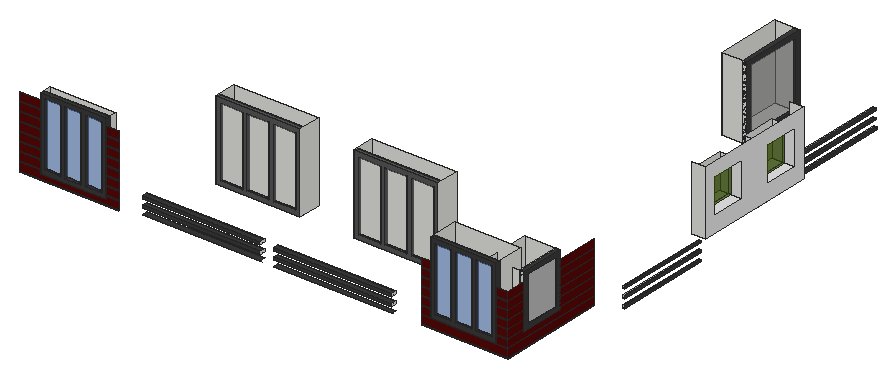
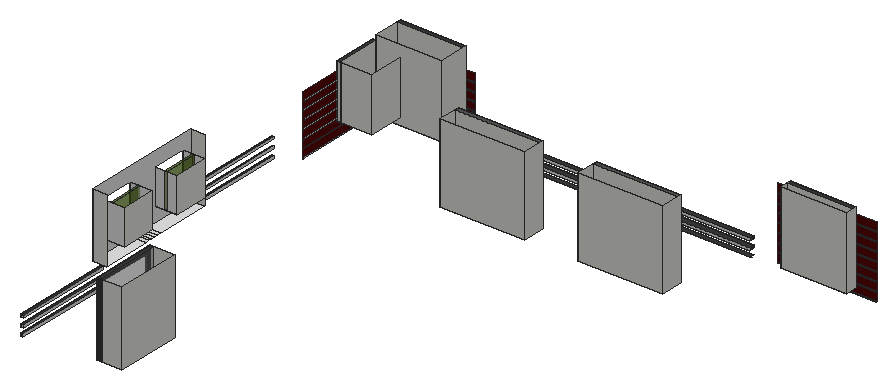
# SketchUp Ruby script. Lengths in inches.
U = 1.inch
M = Sketchup.active_model
def pt(a) = Geom::Point3d.new(a.map { |v| v * U })
def face(e, loops, mat)
  f = e.add_face(loops[0].map { |a| pt(a) })
  loops[1..].each { |l| e.add_face(l.map { |a| pt(a) }).erase! }
  f.material = f.back_material = mat if mat
  f
end
# faces: each face lists its corners as indices into pts; further lists are holes
def faces(e, pts, list, mat = nil) = list.each { |f| face(e, (f[0].is_a?(Array) ? f : [f]).map { |l| l.map { |i| pts[i] } }, mat) }
# xy, xz, yz: faces in a plane at the given z, y or x. An outline is a flat list of corners, or four numbers for a rectangle; further outlines are holes
def ring(l) = l.size == 4 ? [[l[0], l[1]], [l[2], l[1]], [l[2], l[3]], [l[0], l[3]]] : l.each_slice(2).to_a
def flat(e, list, mat, &to3) = list.each { |f| face(e, (f[0].is_a?(Array) ? f : [f]).map { |l| ring(l).map { |u, v| to3.(u, v) } }, mat) }
def xy(e, z, list, mat = nil) = flat(e, list, mat) { |x, y| [x, y, z] }
def xz(e, y, list, mat = nil) = flat(e, list, mat) { |x, z| [x, y, z] }
def yz(e, x, list, mat = nil) = flat(e, list, mat) { |y, z| [x, y, z] }
def lines(e, pts, list) = list.each { |a, b| e.add_line(pt(pts[a]), pt(pts[b])) }
# prism: a flat outline (further loops are holes) pulled along v
def prism(e, loops, v, mat = nil)
  f = face(e, loops, mat); d = Geom::Vector3d.new(v.map { |x| x * U })
  f.pushpull(f.normal.samedirection?(d) ? d.length : -d.length)
end
def box(e, o, s, mat = nil) = prism(e, [[o, [o[0] + s[0], o[1], o[2]], [o[0] + s[0], o[1] + s[1], o[2]], [o[0], o[1] + s[1], o[2]]]], [0, 0, s[2]], mat)
def at(x, y, z, deg = 0) = Geom::Transformation.translation(pt([x, y, z])) * Geom::Transformation.rotation(ORIGIN, Z_AXIS, deg.degrees)
def axes(o, x, y, z) = Geom::Transformation.new([*x, 0, *y, 0, *z, 0, *pt(o).to_a, 1])
def part(name) = M.definitions.add(name)
# library, detail: a bought-in or finely detailed component or shape, given as its bounding box
def library(name, o, s) = part(name).tap { |d| box(d.entities, o, s) }
def detail(e, o, s) = box(e.add_group.entities, o, s)
def put(e, d, t, mat = nil) = e.add_instance(d, t).tap { |i| i.material = mat if mat }
def group(e, t, mat = nil) = e.add_group.tap { |g| g.transformation = t; g.material = mat if mat }.entities
root = M.entities
M.materials.add("Generic").color = [86, 8, 8]
M.materials.add("Generic\#5").color = [230, 230, 230]
M.materials.add("[Color M06]").color = [86, 86, 86]
M.materials.add("[Color M07]").color = [58, 58, 58]
M.materials.add("[Mirror 01]").color = [185, 185, 185]
M.materials.add("[Mirror 02]1").color = [226, 226, 226]
M.materials["[Mirror 02]1"].alpha = 0.26
M.materials.add("[Translucent Glass Blue]").color = [100, 149, 237]
M.materials["[Translucent Glass Blue]"].alpha = 0.5
M.materials.add("[Translucent Glass Dark Green]").color = [62, 91, 5]
M.materials["[Translucent Glass Dark Green]"].alpha = 0.5
M.materials.add("[Translucent Glass Gray]").color = [127, 127, 127]
M.materials["[Translucent Glass Gray]"].alpha = 0.35
c1 = part("Group\#5")
xy(c1.entities,0,[[0,0,6,92.0625]],"[Color M07]")
xy(c1.entities,6.58,[[3,6.58,6,85.48]],"[Color M07]")
xy(c1.entities,96.73,[[3,6.58,6,85.48]],"[Color M07]")
xy(c1.entities,103.3125,[[0,0,6,92.0625]],"[Color M07]")
xz(c1.entities,0,[[0,0,6,103.3125]],"[Color M07]")
xz(c1.entities,6.58,[[3,6.58,6,96.73]],"[Color M07]")
xz(c1.entities,85.48,[[3,6.58,6,96.73]],"[Color M07]")
xz(c1.entities,92.0625,[[0,0,6,103.3125]],"[Color M07]")
yz(c1.entities,0,[[0,0,92.0625,103.3125]],"[Translucent Glass Gray]")
yz(c1.entities,3,[[6.58,6.58,85.48,96.73]],"[Translucent Glass Gray]")
yz(c1.entities,6,[[[0,0,92.0625,103.3125],[6.58,6.58,85.48,96.73]]],"[Color M07]")
c2 = part("Group\#4")
xy(c2.entities,0,[[0,0,117.75,6]],"[Color M06]")
xy(c2.entities,6.37,[[6.37,0,37.125,3],[43.5,0,74.25,3],[80.625,0,111.38,3]],"[Color M06]")
xy(c2.entities,103.75,[[6.37,0,37.125,3],[43.5,0,74.25,3],[80.625,0,111.38,3]],"[Color M06]")
xy(c2.entities,110.125,[[0,0,117.75,6]],"[Color M06]")
xz(c2.entities,0,[[[0,0,117.75,110.125],[6.37,6.37,37.125,103.75],[80.625,6.37,111.38,103.75],[43.5,6.37,74.25,103.75]]],"[Color M06]")
xz(c2.entities,3,[[6.37,6.37,37.125,103.75],[43.5,6.37,74.25,103.75],[80.625,6.37,111.38,103.75]],"[Mirror 02]1")
xz(c2.entities,6,[[0,0,117.75,110.125]])
yz(c2.entities,0,[[0,0,6,110.125]],"[Color M06]")
yz(c2.entities,6.37,[[0,6.37,3,103.75]],"[Color M06]")
yz(c2.entities,37.125,[[0,6.37,3,103.75]],"[Color M06]")
yz(c2.entities,43.5,[[0,6.37,3,103.75]],"[Color M06]")
yz(c2.entities,74.25,[[0,6.37,3,103.75]],"[Color M06]")
yz(c2.entities,80.625,[[0,6.37,3,103.75]],"[Color M06]")
yz(c2.entities,111.38,[[0,6.37,3,103.75]],"[Color M06]")
yz(c2.entities,117.75,[[0,0,6,110.125]],"[Color M06]")
c3 = part("Group\#2")
xy(c3.entities,0,[[0,0,91.6875,6]],"[Color M07]")
xy(c3.entities,6.1,[[6.1,0,28.53,3],[34.63,0,57.06,3],[63.16,0,85.59,3]],"[Color M07]")
xy(c3.entities,95.34,[[6.1,0,28.53,3],[34.63,0,57.06,3],[63.16,0,85.59,3]],"[Color M07]")
xy(c3.entities,101.4375,[[0,0,91.6875,6]],"[Color M07]")
xz(c3.entities,0,[[[0,0,91.6875,101.4375],[34.63,6.1,57.06,95.34],[63.16,6.1,85.59,95.34],[6.1,6.1,28.53,95.34]]],"[Color M07]")
xz(c3.entities,3,[[6.1,6.1,28.53,95.34],[34.63,6.1,57.06,95.34],[63.16,6.1,85.59,95.34]],"[Translucent Glass Blue]")
xz(c3.entities,6,[[0,0,91.6875,101.4375]])
yz(c3.entities,0,[[0,0,6,101.4375]],"[Color M07]")
yz(c3.entities,6.1,[[0,6.1,3,95.34]],"[Color M07]")
yz(c3.entities,28.53,[[0,6.1,3,95.34]],"[Color M07]")
yz(c3.entities,34.63,[[0,6.1,3,95.34]],"[Color M07]")
yz(c3.entities,57.06,[[0,6.1,3,95.34]],"[Color M07]")
yz(c3.entities,63.16,[[0,6.1,3,95.34]],"[Color M07]")
yz(c3.entities,85.59,[[0,6.1,3,95.34]],"[Color M07]")
yz(c3.entities,91.6875,[[0,0,6,101.4375]],"[Color M07]")
c4 = part("Group\#3")
xy(c4.entities,0,[[0,0,6,62.6875]],"[Color M07]")
xy(c4.entities,6.1,[[3,6.1,6,56.59]],"[Color M07]")
xy(c4.entities,69.52,[[3,6.1,6,56.59]],"[Color M07]")
xy(c4.entities,75.625,[[0,0,6,62.6875]],"[Color M07]")
xz(c4.entities,0,[[0,0,6,75.625]],"[Color M07]")
xz(c4.entities,6.1,[[3,6.1,6,69.52]],"[Color M07]")
xz(c4.entities,56.59,[[3,6.1,6,69.52]],"[Color M07]")
xz(c4.entities,62.6875,[[0,0,6,75.625]],"[Color M07]")
yz(c4.entities,0,[[0,0,62.6875,75.625]])
yz(c4.entities,3,[[6.1,6.1,56.59,69.52]],"[Mirror 01]")
yz(c4.entities,6,[[[0,0,62.6875,75.625],[6.1,6.1,56.59,69.52]]],"[Color M07]")
c5 = part("Group\#1")
box(c5.entities,[0,0,0],[3,48.3125,48.3125],"[Translucent Glass Dark Green]")
xy(root,651.9375,[[16.6875,113.625,154.5,113.92]])
xy(root,652.65,[[563.75,654.65,598.75,746.71]])
xy(root,652.9375,[[16.6875,113.625,154.5,113.92]])
xy(root,653.82,[[367.1875,118.5,531.5625,125.9375]],"[Color M07]")
xy(root,654.54,[[183.5625,118.5,347.9375,125.9375]],"[Color M07]")
xy(root,656.21,[[205.11,219.4375,322.86,251.5625],[397.99,219.4375,515.74,251.5625]])
xy(root,656.79,[[723.95,281.625,727.32,413.625]],"[Color M07]")
xy(root,656.83,[[689.08,624.8125,693.27,762.8125]],"[Color M07]")
xy(root,657.48,[[577.6875,113.625,698.4375,113.92],[698.14,113.92,698.4375,263.625]])
xy(root,658.48,[[577.6875,113.625,698.4375,113.92],[698.14,113.92,698.4375,263.625]])
xy(root,659.61,[[44.83,113.625,136.51,130.0625]])
xy(root,659.92,[[723.95,281.625,727.32,413.625]],"[Color M07]")
xy(root,660.15,[[689.08,624.8125,693.27,762.8125]],"[Color M07]")
xy(root,662,[[367.1875,118.5,531.5625,125.9375]],"[Color M07]")
xy(root,662.73,[[183.5625,118.5,347.9375,125.9375]],"[Color M07]")
xy(root,664.4375,[[16.6875,113.625,44.83,113.625,44.83,113.93,16.6875,113.92],[136.51,113.625,154.5,113.625,154.5,113.92,136.51,113.93]])
xy(root,665.4375,[[16.6875,113.625,16.6875,113.92,44.83,113.93,44.83,113.625],[136.51,113.625,136.51,113.93,154.5,113.92,154.5,113.625]])
xy(root,665.82,[[367.1875,118.5,531.5625,125.9375]],"[Color M07]")
xy(root,666.54,[[183.5625,118.5,347.9375,125.9375]],"[Color M07]")
xy(root,668.79,[[723.95,281.625,727.32,413.625]],"[Color M07]")
xy(root,668.8125,[[688.37,624.8125,692.56,762.8125]],"[Color M07]")
xy(root,669.42,[[577.6875,113.625,698.4375,113.92],[698.14,113.92,698.4375,263.625]])
xy(root,669.93,[[589.83,113.93,681.51,156.125]])
xy(root,670.42,[[577.6875,113.625,577.6875,113.92,589.83,113.93,589.83,113.625],[681.51,113.625,681.51,113.93,698.14,113.92,698.4375,113.92,698.4375,113.625],[698.14,113.92,698.4375,263.625]])
xy(root,671.92,[[723.95,281.625,727.32,413.625]],"[Color M07]")
xy(root,672.125,[[688.37,624.8125,692.56,762.8125]],"[Color M07]")
xy(root,672.98,[[698.4375,510.93,717.1875,516.93],[698.4375,516.93,717.1875,521.18],[698.4375,521.18,717.1875,527.18],[698.4375,527.18,717.1875,531.45],[698.4375,531.45,717.1875,537.45]])
xy(root,672.98,[[698.4375,434.68,717.1875,510.93],[698.4375,537.45,717.1875,606.05]],"Generic\#5")
xy(root,674,[[367.1875,118.5,531.5625,125.9375]],"[Color M07]")
xy(root,674.73,[[183.5625,118.5,347.9375,125.9375]],"[Color M07]")
xy(root,676.9375,[[16.6875,113.625,44.83,113.625,44.83,113.93,16.6875,113.92],[136.51,113.625,154.5,113.625,154.5,113.92,136.51,113.93]])
xy(root,677.82,[[367.1875,118.5,531.5625,125.9375]],"[Color M07]")
xy(root,677.9375,[[16.6875,113.625,16.6875,113.92,44.83,113.93,44.83,113.625],[136.51,113.625,136.51,113.93,154.5,113.92,154.5,113.625]])
xy(root,678.54,[[183.5625,118.5,347.9375,125.9375]],"[Color M07]")
xy(root,678.61,[[648.625,141.33,698.4375,204.02]])
xy(root,680.79,[[723.95,281.625,727.32,413.625]],"[Color M07]")
xy(root,680.8125,[[688.37,624.8125,692.56,762.8125]],"[Color M07]")
xy(root,681.37,[[577.6875,113.625,589.83,113.625,589.83,113.93,577.6875,113.92],[681.51,113.625,698.4375,113.625,698.4375,113.92,698.14,113.92,681.51,113.93],[698.14,113.92,698.4375,141.33]])
xy(root,681.72,[[698.14,204.02,698.4375,263.625]])
xy(root,682.37,[[577.6875,113.625,577.6875,113.92,589.83,113.93,589.83,113.625],[681.51,113.625,681.51,113.93,698.14,113.92,698.4375,113.92,698.4375,113.625],[698.14,113.92,698.4375,141.33]])
xy(root,682.72,[[698.14,204.02,698.4375,263.625]])
xy(root,683.92,[[723.95,281.625,727.32,413.625]],"[Color M07]")
xy(root,684.125,[[688.37,624.8125,692.56,762.8125]],"[Color M07]")
xy(root,689.4375,[[16.6875,113.625,44.83,113.92],[136.51,113.625,154.5,113.92]])
xy(root,690.4375,[[16.6875,113.625,44.83,113.92],[136.51,113.625,154.5,113.92]])
xy(root,693.31,[[698.14,113.625,698.4375,141.33]])
xy(root,693.3125,[[577.6875,113.625,589.83,113.92],[681.51,113.625,698.14,113.92]])
xy(root,693.62,[[698.14,204.02,698.4375,263.625]])
xy(root,694.3125,[[577.6875,113.625,589.83,113.92],[681.51,113.625,698.4375,113.92],[698.14,113.92,698.4375,141.33]])
xy(root,694.62,[[698.14,204.02,698.4375,263.625]])
xy(root,695.24,[[685.875,449.87,717.1875,498.18],[685.875,541.87,717.1875,590.18]],"Generic\#5")
xy(root,701.9375,[[16.6875,113.625,44.83,113.92],[136.51,113.625,154.5,113.92]])
xy(root,702.9375,[[16.6875,113.625,44.83,113.92],[136.51,113.625,154.5,113.92]])
xy(root,705.26,[[577.6875,113.625,589.83,113.92],[681.51,113.625,698.4375,113.92],[698.14,113.92,698.4375,141.33]])
xy(root,705.52,[[698.14,204.02,698.4375,263.625]])
xy(root,706.26,[[577.6875,113.625,589.83,113.92],[681.51,113.625,698.4375,113.92],[698.14,113.92,698.4375,141.33]])
xy(root,706.52,[[698.14,204.02,698.4375,263.625]])
xy(root,714.4375,[[16.6875,113.625,44.83,113.92],[136.51,113.625,154.5,113.92]])
xy(root,715.4375,[[16.6875,113.625,44.83,113.92],[136.51,113.625,154.5,113.92]])
xy(root,717.21,[[577.6875,113.625,589.83,113.92],[681.51,113.625,698.4375,113.92],[698.14,113.92,698.4375,141.33]])
xy(root,717.43,[[698.14,204.02,698.4375,263.625]])
xy(root,718.21,[[577.6875,113.625,589.83,113.92],[681.51,113.625,698.4375,113.92],[698.14,113.92,698.4375,141.33]])
xy(root,718.43,[[698.14,204.02,698.4375,263.625]])
xy(root,726.9375,[[16.6875,113.625,44.83,113.92],[136.51,113.625,154.5,113.92]])
xy(root,727.9375,[[16.6875,113.625,44.83,113.92],[136.51,113.625,154.5,113.92]])
xy(root,729.15,[[577.6875,113.625,589.83,113.92],[681.51,113.625,698.4375,113.92],[698.14,113.92,698.4375,141.33]])
xy(root,729.33,[[698.14,204.02,698.4375,263.625]])
xy(root,730.15,[[577.6875,113.625,589.83,113.92],[681.51,113.625,698.4375,113.92],[698.14,113.92,698.4375,141.33]])
xy(root,730.33,[[698.14,204.02,698.4375,263.625]])
xy(root,739.4375,[[16.6875,113.625,44.83,113.625,44.83,113.93,16.6875,113.92],[136.51,113.625,154.5,113.625,154.5,113.92,136.51,113.93]])
xy(root,740.4375,[[16.6875,113.625,16.6875,113.92,44.83,113.93,44.83,113.625],[136.51,113.625,136.51,113.93,154.5,113.92,154.5,113.625]])
xz(root,113.625,[[16.6875,652.9375,154.5,652.9375,154.5,664.4375,136.51,664.4375,136.51,659.61,44.83,659.61,44.83,664.4375,16.6875,664.4375],[577.6875,658.48,698.4375,669.42],[16.6875,665.4375,44.83,676.9375],[136.51,665.4375,154.5,676.9375],[577.6875,670.42,589.83,681.37],
  [681.51,670.42,698.4375,681.37],[16.6875,677.9375,44.83,689.4375],[136.51,677.9375,154.5,689.4375],[577.6875,682.37,589.83,693.3125],[681.51,682.37,698.4375,682.37,698.4375,693.31,698.14,693.31,698.14,693.3125,681.51,693.3125],
  [16.6875,690.4375,44.83,701.9375],[136.51,690.4375,154.5,701.9375],[577.6875,694.3125,589.83,705.26],[681.51,694.3125,698.4375,705.26],[16.6875,702.9375,44.83,714.4375],
  [136.51,702.9375,154.5,714.4375],[577.6875,706.26,589.83,717.21],[681.51,706.26,698.4375,717.21],[16.6875,715.4375,44.83,726.9375],[136.51,715.4375,154.5,726.9375],
  [577.6875,718.21,589.83,729.15],[681.51,718.21,698.4375,729.15],[16.6875,727.9375,44.83,739.4375],[136.51,727.9375,154.5,739.4375],[577.6875,730.15,589.83,741.1],
  [681.51,730.15,698.4375,741.1],[16.6875,740.4375,44.83,751.9375],[136.51,740.4375,154.5,751.9375]],"Generic")
xz(root,113.92,[[16.6875,651.9375,154.5,652.9375],[577.6875,657.48,698.14,658.48],[16.6875,689.4375,44.83,690.4375],[136.51,689.4375,154.5,690.4375],[577.6875,693.3125,589.83,694.3125],
  [681.51,693.3125,698.14,694.3125],[16.6875,701.9375,44.83,702.9375],[136.51,701.9375,154.5,702.9375],[577.6875,705.26,589.83,706.26],[681.51,705.26,698.14,706.26],
  [16.6875,714.4375,44.83,715.4375],[136.51,714.4375,154.5,715.4375],[577.6875,717.21,589.83,718.21],[681.51,717.21,698.14,718.21],[16.6875,726.9375,44.83,727.9375],
  [136.51,726.9375,154.5,727.9375],[577.6875,729.15,589.83,730.15],[681.51,729.15,698.14,730.15]])
xz(root,118.5,[[367.1875,662,531.5625,665.82],[183.5625,662.73,347.9375,666.54],[367.1875,674,531.5625,677.82],[183.5625,674.73,347.9375,678.54]],"[Color M07]")
xz(root,125.9375,[[367.1875,662,531.5625,665.82],[183.5625,662.73,347.9375,666.54],[367.1875,674,531.5625,677.82],[183.5625,674.73,347.9375,678.54]])
xz(root,130.0625,[[44.83,659.61,136.51,761.05]])
xz(root,141.33,[[648.625,678.61,648.625,754.24,698.4375,754.24,698.4375,754.05,698.14,754.05,698.14,753.05,698.4375,753.05,698.4375,742.11,698.14,742.11,698.14,741.1,698.4375,741.1,698.4375,730.15,698.14,730.15,698.14,729.15,698.4375,729.15,698.4375,718.21,698.14,718.21,698.14,717.21,698.4375,717.21,698.4375,706.26,698.14,706.26,698.14,705.26,698.4375,705.26,698.4375,694.3125,698.14,694.3125,698.14,693.31,698.4375,693.31,698.4375,682.37,698.14,682.37,698.14,681.37,698.4375,681.37,698.4375,678.61]])
xz(root,156.125,[[589.83,669.93,681.51,771.36]])
xz(root,204.02,[[648.625,678.61,698.4375,678.61,698.4375,681.72,698.14,681.72,698.14,682.72,698.4375,682.72,698.4375,693.62,698.14,693.62,698.14,694.62,698.4375,694.62,698.4375,705.52,698.14,705.52,698.14,706.52,698.4375,706.52,698.4375,717.43,698.14,717.43,698.14,718.43,698.4375,718.43,698.4375,729.33,698.14,729.33,698.14,730.33,698.4375,730.33,698.4375,741.23,698.14,741.23,698.14,742.23,698.4375,742.23,698.4375,753.13,698.14,753.13,698.14,754.13,698.4375,754.13,698.4375,754.24,648.625,754.24]])
xz(root,251.5625,[[205.11,656.21,322.86,766.34],[397.99,656.21,515.74,766.34]])
xz(root,263.625,[[698.14,657.48,698.4375,658.48],[698.14,669.42,698.4375,670.42],[698.14,681.72,698.4375,682.72],[698.14,693.62,698.4375,694.62],[698.14,705.52,698.4375,706.52],
  [698.14,717.43,698.4375,718.43],[698.14,729.33,698.4375,730.33]])
xz(root,413.625,[[723.95,656.79,727.32,659.92],[723.95,668.79,727.32,671.92],[723.95,680.79,727.32,683.92]])
xz(root,434.68,[[698.4375,672.98,717.1875,762.91]])
xz(root,449.87,[[685.875,695.24,717.1875,743.55]],"Generic\#5")
xz(root,498.18,[[685.875,695.24,717.1875,743.55]],"Generic\#5")
xz(root,541.87,[[685.875,695.24,717.1875,743.55]],"Generic\#5")
xz(root,590.18,[[685.875,695.24,717.1875,743.55]],"Generic\#5")
xz(root,606.05,[[698.4375,672.98,717.1875,762.91]])
xz(root,654.65,[[563.75,652.65,598.75,755.96]])
xz(root,746.71,[[563.75,652.65,598.75,755.96]])
xz(root,762.8125,[[689.08,656.83,693.27,660.15],[688.37,668.8125,692.56,672.125],[688.37,680.8125,692.56,684.125]])
yz(root,44.83,[[113.625,659.61,130.0625,659.61,130.0625,761.05,113.625,761.05,113.625,752.9375,113.93,752.9375,113.93,751.9375,113.625,751.9375,113.625,740.4375,113.93,740.4375,113.93,739.4375,113.625,739.4375,113.625,727.9375,113.92,727.9375,113.92,726.9375,113.625,726.9375,113.625,715.4375,113.92,715.4375,113.92,714.4375,113.625,714.4375,113.625,702.9375,113.92,702.9375,113.92,701.9375,113.625,701.9375,113.625,690.4375,113.92,690.4375,113.92,689.4375,113.625,689.4375,113.625,677.9375,113.93,677.9375,113.93,676.9375,113.625,676.9375,113.625,665.4375,113.93,665.4375,113.93,664.4375,113.625,664.4375]])
yz(root,136.51,[[113.625,659.61,113.625,664.4375,113.93,664.4375,113.93,665.4375,113.625,665.4375,113.625,676.9375,113.93,676.9375,113.93,677.9375,113.625,677.9375,113.625,689.4375,113.92,689.4375,113.92,690.4375,113.625,690.4375,113.625,701.9375,113.92,701.9375,113.92,702.9375,113.625,702.9375,113.625,714.4375,113.92,714.4375,113.92,715.4375,113.625,715.4375,113.625,726.9375,113.92,726.9375,113.92,727.9375,113.625,727.9375,113.625,739.4375,113.93,739.4375,113.93,740.4375,113.625,740.4375,113.625,751.9375,113.93,751.9375,113.93,752.9375,113.625,752.9375,113.625,761.05,130.0625,761.05,130.0625,659.61]])
yz(root,154.5,[[113.625,651.9375,113.92,652.9375],[113.625,664.4375,113.92,665.4375],[113.625,676.9375,113.92,677.9375],[113.625,689.4375,113.92,690.4375],[113.625,701.9375,113.92,702.9375],
  [113.625,714.4375,113.92,715.4375],[113.625,726.9375,113.92,727.9375],[113.625,739.4375,113.92,740.4375]])
yz(root,205.11,[[219.4375,656.21,251.5625,766.34]])
yz(root,322.86,[[219.4375,656.21,251.5625,766.34]])
yz(root,347.9375,[[118.5,662.73,125.9375,666.54],[118.5,674.73,125.9375,678.54]])
yz(root,397.99,[[219.4375,656.21,251.5625,766.34]])
yz(root,515.74,[[219.4375,656.21,251.5625,766.34]])
yz(root,531.5625,[[118.5,662,125.9375,665.82],[118.5,674,125.9375,677.82]])
yz(root,563.75,[[654.65,652.65,746.71,755.96]])
yz(root,577.6875,[[113.625,657.48,113.92,658.48],[113.625,669.42,113.92,670.42],[113.625,681.37,113.92,682.37],[113.625,693.3125,113.92,694.3125],[113.625,705.26,113.92,706.26],
  [113.625,717.21,113.92,718.21],[113.625,729.15,113.92,730.15]])
yz(root,589.83,[[113.93,669.93,156.125,669.93,156.125,771.36,113.625,771.36,113.625,765.99,113.93,765.99,113.93,764.99,113.625,764.99,113.625,754.05,113.93,754.05,113.93,753.05,113.625,753.05,113.625,742.1,113.92,742.1,113.92,741.1,113.625,741.1,113.625,730.15,113.92,730.15,113.92,729.15,113.625,729.15,113.625,718.21,113.92,718.21,113.92,717.21,113.625,717.21,113.625,706.26,113.92,706.26,113.92,705.26,113.625,705.26,113.625,694.3125,113.92,694.3125,113.92,693.3125,113.625,693.3125,113.625,682.37,113.93,682.37,113.93,681.37,113.625,681.37,113.625,670.42,113.93,670.42]])
yz(root,648.625,[[141.33,678.61,204.02,754.24]])
yz(root,681.51,[[113.93,669.93,113.93,670.42,113.625,670.42,113.625,681.37,113.93,681.37,113.93,682.37,113.625,682.37,113.625,693.3125,113.92,693.3125,113.92,694.3125,113.625,694.3125,113.625,705.26,113.92,705.26,113.92,706.26,113.625,706.26,113.625,717.21,113.92,717.21,113.92,718.21,113.625,718.21,113.625,729.15,113.92,729.15,113.92,730.15,113.625,730.15,113.625,741.1,113.92,741.1,113.92,742.1,113.625,742.1,113.625,753.05,113.93,753.05,113.93,754.05,113.625,754.05,113.625,764.99,113.93,764.99,113.93,765.99,113.625,765.99,113.625,771.36,156.125,771.36,156.125,669.93]])
yz(root,685.875,[[449.87,695.24,498.18,743.55],[541.87,695.24,590.18,743.55]])
yz(root,688.37,[[624.8125,668.8125,762.8125,672.125],[624.8125,680.8125,762.8125,684.125]])
yz(root,689.08,[[624.8125,656.83,762.8125,660.15]])
yz(root,692.56,[[624.8125,668.8125,762.8125,672.125],[624.8125,680.8125,762.8125,684.125]],"[Color M07]")
yz(root,693.27,[[624.8125,656.83,762.8125,660.15]],"[Color M07]")
yz(root,698.14,[[113.92,657.48,263.625,658.48],[113.92,669.42,263.625,670.42],[113.92,681.37,141.33,682.37],[204.02,681.72,263.625,682.72],[113.625,693.31,141.33,693.31,141.33,694.3125,113.92,694.3125,113.92,693.3125,113.625,693.3125],
  [204.02,693.62,263.625,694.62],[113.92,705.26,141.33,706.26],[204.02,705.52,263.625,706.52],[113.92,717.21,141.33,718.21],[204.02,717.43,263.625,718.43],
  [113.92,729.15,141.33,730.15],[204.02,729.33,263.625,730.33]])
yz(root,698.4375,[[113.625,658.48,263.625,669.42],[113.625,670.42,263.625,670.42,263.625,681.72,204.02,681.72,204.02,678.61,141.33,678.61,141.33,681.37,113.625,681.37],[113.625,682.37,141.33,693.31],[204.02,682.72,263.625,693.62],[113.625,694.3125,141.33,705.26],
  [204.02,694.62,263.625,705.52],[113.625,706.26,141.33,717.21],[204.02,706.52,263.625,717.43],[113.625,718.21,141.33,729.15],[204.02,718.43,263.625,729.33],
  [113.625,730.15,141.33,741.1],[204.02,730.33,263.625,741.23]],"Generic")
yz(root,717.1875,[[[434.68,672.98,606.05,762.91],[449.87,695.24,498.18,743.55],[541.87,695.24,590.18,743.55]]],"Generic\#5")
yz(root,723.95,[[281.625,656.79,413.625,659.92],[281.625,668.79,413.625,671.92],[281.625,680.79,413.625,683.92]])
yz(root,727.32,[[281.625,656.79,413.625,659.92],[281.625,668.79,413.625,671.92],[281.625,680.79,413.625,683.92]],"[Color M07]")
p = [[16.6875,113.92,664.4375],[44.83,113.93,664.4375],[44.83,113.93,665.4375],[16.6875,113.92,665.4375],[154.5,113.92,664.4375],[154.5,113.92,665.4375],
  [136.51,113.93,665.4375],[136.51,113.93,664.4375],[589.83,113.93,669.93],[589.83,113.93,670.42],[577.6875,113.92,670.42],[577.6875,113.92,669.42],
  [698.14,113.92,669.42],[698.14,113.92,670.42],[681.51,113.93,670.42],[681.51,113.93,669.93],[16.6875,113.92,676.9375],[44.83,113.93,676.9375],
  [44.83,113.93,677.9375],[16.6875,113.92,677.9375],[154.5,113.92,676.9375],[154.5,113.92,677.9375],[136.51,113.93,677.9375],[136.51,113.93,676.9375],
  [589.83,113.93,681.37],[589.83,113.93,682.37],[577.6875,113.92,682.37],[577.6875,113.92,681.37],[698.14,113.92,682.37],[681.51,113.93,682.37],
  [681.51,113.93,681.37],[698.14,113.92,681.37],[16.6875,113.92,739.4375],[44.83,113.93,739.4375],[44.83,113.93,740.4375],[16.6875,113.92,740.4375],
  [154.5,113.92,739.4375],[154.5,113.92,740.4375],[136.51,113.93,740.4375],[136.51,113.93,739.4375],[531.5625,121.625,651.9375],[367.1875,121.625,651.9375],
  [531.5625,121.625,663.9375],[367.1875,121.625,663.9375],[531.5625,121.625,675.9375],[367.1875,121.625,675.9375],[347.9375,121.625,651.9375],[183.5625,121.625,651.9375],
  [347.9375,121.625,663.9375],[183.5625,121.625,663.9375],[347.9375,121.625,675.9375],[183.5625,121.625,675.9375],[691.4375,762.8125,657.9375],[691.4375,624.8125,657.9375],
  [691.4375,762.8125,669.9375],[691.4375,624.8125,669.9375],[691.4375,762.8125,681.9375],[691.4375,624.8125,681.9375],[726,413.625,657.9375],[726,281.625,657.9375],
  [726,413.625,669.9375],[726,281.625,669.9375],[726,413.625,681.9375],[726,281.625,681.9375]]
faces(root,p,[[0,1,2,3],[4,5,6,7],[8,9,10,11,12,13,14,15],[16,17,18,19],[20,21,22,23],[24,25,26,27],[28,29,30,31],[32,33,34,35],
  [36,37,38,39]])
lines(root,p,[[40,41],[42,43],[44,45],[46,47],[48,49],[50,51],[52,53],[54,55],[56,57],[58,59],[60,61],[62,63]])
put(root,c1,at(592.75,654.65,652.65))
put(root,c2,at(205.11,219.4375,656.21))
put(root,c2,at(397.99,219.4375,656.21))
put(root,c3,at(44.83,113.625,659.61))
put(root,c3,at(589.83,113.625,669.93))
put(root,c4,at(692.4375,141.33,678.61))
put(root,c5,at(702.4375,540.12,695.24))
put(root,c5,at(699.4375,449.87,695.24))
